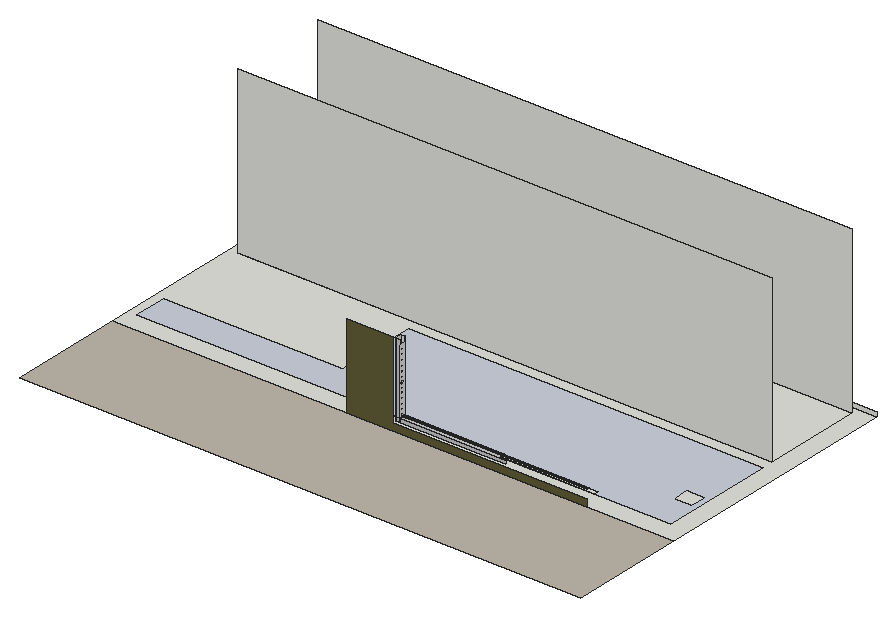
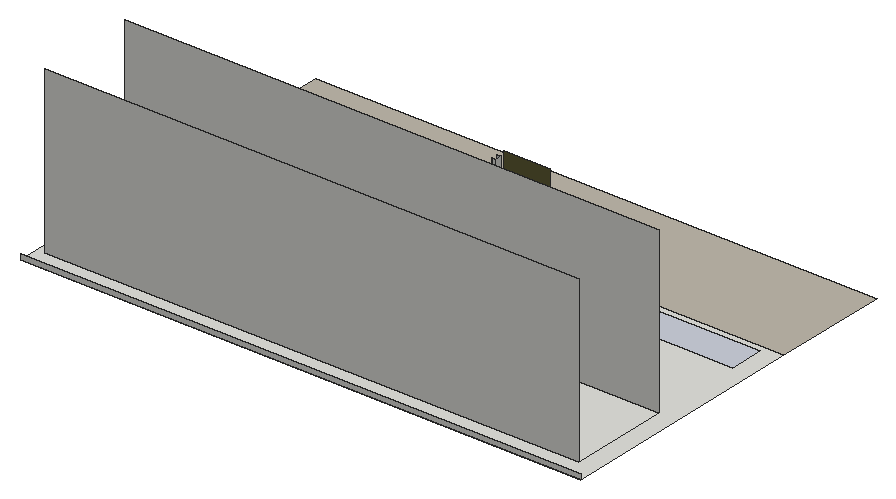
# SketchUp Ruby script. Lengths in inches.
U = 1.inch
M = Sketchup.active_model
def pt(a) = Geom::Point3d.new(a.map { |v| v * U })
def face(e, loops, mat)
  f = e.add_face(loops[0].map { |a| pt(a) })
  loops[1..].each { |l| e.add_face(l.map { |a| pt(a) }).erase! }
  f.material = f.back_material = mat if mat
  f
end
# faces: each face lists its corners as indices into pts; further lists are holes
def faces(e, pts, list, mat = nil) = list.each { |f| face(e, (f[0].is_a?(Array) ? f : [f]).map { |l| l.map { |i| pts[i] } }, mat) }
# xy, xz, yz: faces in a plane at the given z, y or x. An outline is a flat list of corners, or four numbers for a rectangle; further outlines are holes
def ring(l) = l.size == 4 ? [[l[0], l[1]], [l[2], l[1]], [l[2], l[3]], [l[0], l[3]]] : l.each_slice(2).to_a
def flat(e, list, mat, &to3) = list.each { |f| face(e, (f[0].is_a?(Array) ? f : [f]).map { |l| ring(l).map { |u, v| to3.(u, v) } }, mat) }
def xy(e, z, list, mat = nil) = flat(e, list, mat) { |x, y| [x, y, z] }
def xz(e, y, list, mat = nil) = flat(e, list, mat) { |x, z| [x, y, z] }
def yz(e, x, list, mat = nil) = flat(e, list, mat) { |y, z| [x, y, z] }
def lines(e, pts, list) = list.each { |a, b| e.add_line(pt(pts[a]), pt(pts[b])) }
# prism: a flat outline (further loops are holes) pulled along v
def prism(e, loops, v, mat = nil)
  f = face(e, loops, mat); d = Geom::Vector3d.new(v.map { |x| x * U })
  f.pushpull(f.normal.samedirection?(d) ? d.length : -d.length)
end
def box(e, o, s, mat = nil) = prism(e, [[o, [o[0] + s[0], o[1], o[2]], [o[0] + s[0], o[1] + s[1], o[2]], [o[0], o[1] + s[1], o[2]]]], [0, 0, s[2]], mat)
def at(x, y, z, deg = 0) = Geom::Transformation.translation(pt([x, y, z])) * Geom::Transformation.rotation(ORIGIN, Z_AXIS, deg.degrees)
def axes(o, x, y, z) = Geom::Transformation.new([*x, 0, *y, 0, *z, 0, *pt(o).to_a, 1])
def part(name) = M.definitions.add(name)
# library, detail: a bought-in or finely detailed component or shape, given as its bounding box
def library(name, o, s) = part(name).tap { |d| box(d.entities, o, s) }
def detail(e, o, s) = box(e.add_group.entities, o, s)
def put(e, d, t, mat = nil) = e.add_instance(d, t).tap { |i| i.material = mat if mat }
def group(e, t, mat = nil) = e.add_group.tap { |g| g.transformation = t; g.material = mat if mat }.entities
root = M.entities
M.materials.add("[0057_DarkKhaki]").color = [96, 93, 54]
M.materials.add("[Cinder Block]").color = [191, 184, 171]
M.materials.add("[Marble Carrara Floor Tile]").color = [204, 208, 219]
M.materials.add("[Polished Concrete New]").color = [200, 200, 203]
M.materials.add("[Polished Concrete Old]").color = [229, 229, 229]
xy(root,0,[[11.875,223.5,1099.23,714.96]])
xy(root,0,[[11.875,0,1099.23,223.5]],"[Cinder Block]")
xy(root,9,[[38.27,494.96,1072.84,688.57]])
xy(root,9,[[[38.27,249.9,1072.84,249.9,1072.84,472.99,386.67,472.99,386.67,314.12,38.27,314.12],[1027.11,314.12,1062.63,346.6]]],"[Marble Carrara Floor Tile]")
xy(root,14.9375,[[748.36,230.28,727.92,230.3,727.92,243.88,748.38,243.86],[727.92,230.3,555.05,230.47,562.43,230.47,562.43,244.04,727.92,243.88],[555.05,230.47,562.43,230.47,562.43,244.04,555.05,244.05],[931.07,243.6875,931.07,249.9,555.05,249.9,555.05,244.05,562.43,244.05,562.43,244.04,727.92,243.88,748.38,243.86,768.82,243.84],[562.43,244.04,555.05,244.05,562.43,244.05]])
xy(root,21,[[754.67,230.27,754.67,243.86,748.38,243.86,727.92,243.88,562.43,244.04,562.43,230.47,555.05,230.47]],"[Polished Concrete New]")
xz(root,223.5,[[465.4375,0,931.03,0,931.03,14.9375,555.05,14.9375,555.05,163.5625,465.4375,163.5625]],"[0057_DarkKhaki]")
xz(root,230.47,[[555.05,14.9375,562.43,21]])
xz(root,230.47,[[555.05,21,562.43,158]],"[Polished Concrete New]")
xz(root,244.05,[[555.05,14.9375,562.43,158.26]])
xz(root,494.96,[[38.27,9,1072.84,328.125]])
xz(root,688.57,[[38.27,9,1072.84,328.125]])
xz(root,714.96,[[11.875,0,1099.23,9]])
yz(root,555.05,[[230.47,14.9375,244.05,158.26]])
yz(root,562.43,[[230.47,14.9375,244.04,21],[[244.04,14.9375,244.05,14.9375,244.05,158.26,243.6875,158.26,243.6875,149.47,230.47,149.47,230.47,21,244.04,21],[236.62,77.51,235.53,77.65,234.52,78.07,233.66,78.74,232.99,79.6,232.57,80.61,232.43,81.7,232.57,82.78,232.99,83.79,233.66,84.66,234.52,85.32,235.53,85.74,236.62,85.89,237.7,85.74,238.71,85.32,239.58,84.66,240.24,83.79,240.66,82.78,240.81,81.7,240.66,80.61,240.24,79.6,239.58,78.74,238.71,78.07,237.7,77.65],[236.71,138.15,236.08,138.24,235.5,138.48,234.99,138.87,234.6,139.375,234.36,139.96,234.28,140.59,234.36,141.22,234.6,141.8125,234.99,142.32,235.5,142.7,236.08,142.95,236.71,143.03,237.35,142.95,237.93,142.7,238.4375,142.32,238.83,141.8125,239.07,141.22,239.15,140.59,239.07,139.96,238.83,139.375,238.4375,138.87,237.93,138.48,237.35,138.24],[236.71,129.34,236.08,129.43,235.5,129.67,234.99,130.06,234.6,130.5625,234.36,131.15,234.28,131.78,234.36,132.41,234.6,133,234.99,133.5,235.5,133.89,236.08,134.13,236.71,134.22,237.35,134.13,237.93,133.89,238.4375,133.5,238.83,133,239.07,132.41,239.15,131.78,239.07,131.15,238.83,130.5625,238.4375,130.06,237.93,129.67,237.35,129.43],[236.71,118.53,236.08,118.61,235.5,118.86,234.99,119.24,234.6,119.75,234.36,120.34,234.28,120.97,234.36,121.6,234.6,122.1875,234.99,122.69,235.5,123.08,236.08,123.32,236.71,123.4,237.35,123.32,237.93,123.08,238.4375,122.69,238.83,122.1875,239.07,121.6,239.15,120.97,239.07,120.34,238.83,119.75,238.4375,119.24,237.93,118.86,237.35,118.61],[236.71,108.15,236.08,108.24,235.5,108.48,234.99,108.87,234.6,109.375,234.36,109.96,234.28,110.59,234.36,111.22,234.6,111.8125,234.99,112.32,235.5,112.7,236.08,112.95,236.71,113.03,237.35,112.95,237.93,112.7,238.4375,112.32,238.83,111.8125,239.07,111.22,239.15,110.59,239.07,109.96,238.83,109.375,238.4375,108.87,237.93,108.48,237.35,108.24],[236.71,98.28,236.08,98.36,235.5,98.61,234.99,98.99,234.6,99.5,234.36,100.09,234.28,100.72,234.36,101.35,234.6,101.9375,234.99,102.44,235.5,102.83,236.08,103.07,236.71,103.15,237.35,103.07,237.93,102.83,238.4375,102.44,238.83,101.9375,239.07,101.35,239.15,100.72,239.07,100.09,238.83,99.5,238.4375,98.99,237.93,98.61,237.35,98.36],[236.71,89.28,236.08,89.36,235.5,89.61,234.99,89.99,234.6,90.5,234.36,91.09,234.28,91.72,234.36,92.35,234.6,92.9375,234.99,93.44,235.5,93.83,236.08,94.07,236.71,94.15,237.35,94.07,237.93,93.83,238.4375,93.44,238.83,92.9375,239.07,92.35,239.15,91.72,239.07,91.09,238.83,90.5,238.4375,89.99,237.93,89.61,237.35,89.36],[236.71,70.22,236.08,70.3,235.5,70.54,234.99,70.93,234.6,71.4375,234.36,72.02,234.28,72.65,234.36,73.29,234.6,73.875,234.99,74.38,235.5,74.77,236.08,75.01,236.71,75.09,237.35,75.01,237.93,74.77,238.4375,74.38,238.83,73.875,239.07,73.29,239.15,72.65,239.07,72.02,238.83,71.4375,238.4375,70.93,237.93,70.54,237.35,70.3],[236.71,61.84,236.08,61.93,235.5,62.17,234.99,62.56,234.6,63.0625,234.36,63.65,234.28,64.28,234.36,64.91,234.6,65.5,234.99,66,235.5,66.39,236.08,66.63,236.71,66.72,237.35,66.63,237.93,66.39,238.4375,66,238.83,65.5,239.07,64.91,239.15,64.28,239.07,63.65,238.83,63.0625,238.4375,62.56,237.93,62.17,237.35,61.93],[236.71,52.03,236.08,52.11,235.5,52.36,234.99,52.74,234.6,53.25,234.36,53.84,234.28,54.47,234.36,55.1,234.6,55.6875,234.99,56.19,235.5,56.58,236.08,56.82,236.71,56.9,237.35,56.82,237.93,56.58,238.4375,56.19,238.83,55.6875,239.07,55.1,239.15,54.47,239.07,53.84,238.83,53.25,238.4375,52.74,237.93,52.36,237.35,52.11],[236.71,41.84,236.08,41.93,235.5,42.17,234.99,42.56,234.6,43.0625,234.36,43.65,234.28,44.28,234.36,44.91,234.6,45.5,234.99,46,235.5,46.39,236.08,46.63,236.71,46.72,237.35,46.63,237.93,46.39,238.4375,46,238.83,45.5,239.07,44.91,239.15,44.28,239.07,43.65,238.83,43.0625,238.4375,42.56,237.93,42.17,237.35,41.93],[236.71,23.9,236.08,23.99,235.5,24.23,234.99,24.62,234.6,25.125,234.36,25.71,234.28,26.34,234.36,26.97,234.6,27.5625,234.99,28.07,235.5,28.45,236.08,28.7,236.71,28.78,237.35,28.7,237.93,28.45,238.4375,28.07,238.83,27.5625,239.07,26.97,239.15,26.34,239.07,25.71,238.83,25.125,238.4375,24.62,237.93,24.23,237.35,23.99],[236.71,33.4,236.08,33.49,235.5,33.73,234.99,34.12,234.6,34.625,234.36,35.21,234.28,35.84,234.36,36.47,234.6,37.0625,234.99,37.57,235.5,37.95,236.08,38.2,236.71,38.28,237.35,38.2,237.93,37.95,238.4375,37.57,238.83,37.0625,239.07,36.47,239.15,35.84,239.07,35.21,238.83,34.625,238.4375,34.12,237.93,33.73,237.35,33.49]]])
p = [[768.81,230.26,14.9375],[768.81,230.26,21],[764.33,230.27,21],[754.67,230.27,21],[555.05,230.47,21],[555.05,230.47,14.9375],
  [727.92,230.3,14.9375],[748.36,230.28,14.9375],[727.92,243.88,14.9375],[562.43,244.04,14.9375],[562.43,244.04,21],[727.92,243.88,21],
  [748.38,243.86,14.9375],[748.38,243.86,21],[922.51,236.71,23.9],[922.51,236.08,23.99],[562.43,236.08,23.99],[562.43,236.71,23.9],
  [922.51,237.35,23.99],[562.43,237.35,23.99],[922.51,235.5,24.23],[562.43,235.5,24.23],[922.51,237.93,24.23],[562.43,237.93,24.23],
  [922.51,234.99,24.62],[562.43,234.99,24.62],[922.51,238.4375,24.62],[562.43,238.4375,24.62]]
faces(root,p,[[0,1,2,3,4,5,6,7]],"[Polished Concrete New]")
faces(root,p,[[1,2,3,4,5,6,7,0],[8,9,10,11],[12,8,11,13]])
faces(root,p,[[14,15,16,17],[18,14,17,19],[15,20,21,16],[22,18,19,23],[20,24,25,21],[26,22,23,27]],"[Polished Concrete Old]")
